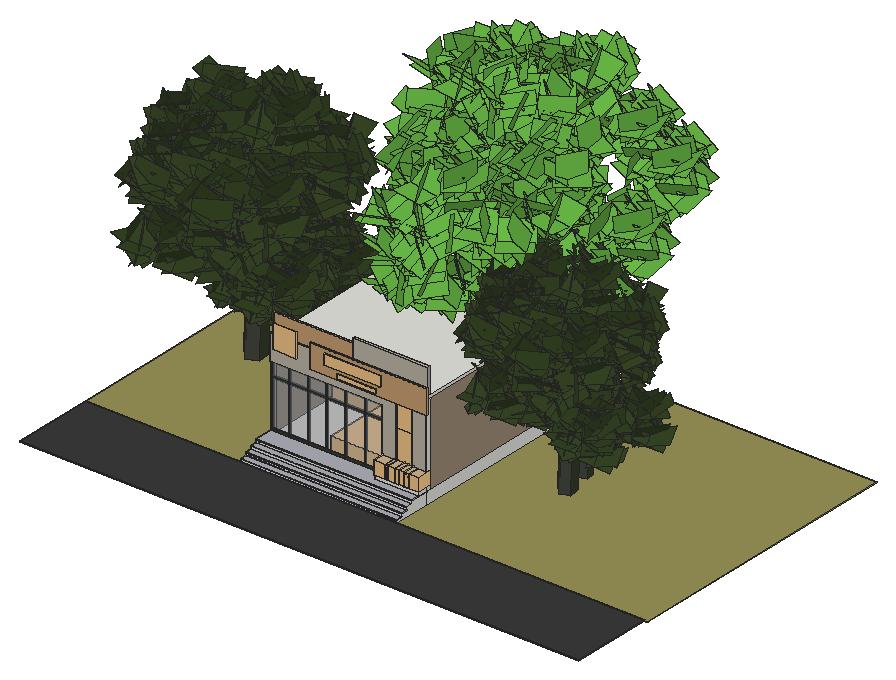
# SketchUp Ruby script. Lengths in inches.
U = 1.inch
M = Sketchup.active_model
def pt(a) = Geom::Point3d.new(a.map { |v| v * U })
def face(e, loops, mat)
  f = e.add_face(loops[0].map { |a| pt(a) })
  loops[1..].each { |l| e.add_face(l.map { |a| pt(a) }).erase! }
  f.material = f.back_material = mat if mat
  f
end
# faces: each face lists its corners as indices into pts; further lists are holes
def faces(e, pts, list, mat = nil) = list.each { |f| face(e, (f[0].is_a?(Array) ? f : [f]).map { |l| l.map { |i| pts[i] } }, mat) }
# xy, xz, yz: faces in a plane at the given z, y or x. An outline is a flat list of corners, or four numbers for a rectangle; further outlines are holes
def ring(l) = l.size == 4 ? [[l[0], l[1]], [l[2], l[1]], [l[2], l[3]], [l[0], l[3]]] : l.each_slice(2).to_a
def flat(e, list, mat, &to3) = list.each { |f| face(e, (f[0].is_a?(Array) ? f : [f]).map { |l| ring(l).map { |u, v| to3.(u, v) } }, mat) }
def xy(e, z, list, mat = nil) = flat(e, list, mat) { |x, y| [x, y, z] }
def xz(e, y, list, mat = nil) = flat(e, list, mat) { |x, z| [x, y, z] }
def yz(e, x, list, mat = nil) = flat(e, list, mat) { |y, z| [x, y, z] }
def lines(e, pts, list) = list.each { |a, b| e.add_line(pt(pts[a]), pt(pts[b])) }
# prism: a flat outline (further loops are holes) pulled along v
def prism(e, loops, v, mat = nil)
  f = face(e, loops, mat); d = Geom::Vector3d.new(v.map { |x| x * U })
  f.pushpull(f.normal.samedirection?(d) ? d.length : -d.length)
end
def box(e, o, s, mat = nil) = prism(e, [[o, [o[0] + s[0], o[1], o[2]], [o[0] + s[0], o[1] + s[1], o[2]], [o[0], o[1] + s[1], o[2]]]], [0, 0, s[2]], mat)
def at(x, y, z, deg = 0) = Geom::Transformation.translation(pt([x, y, z])) * Geom::Transformation.rotation(ORIGIN, Z_AXIS, deg.degrees)
def axes(o, x, y, z) = Geom::Transformation.new([*x, 0, *y, 0, *z, 0, *pt(o).to_a, 1])
def part(name) = M.definitions.add(name)
# library, detail: a bought-in or finely detailed component or shape, given as its bounding box
def library(name, o, s) = part(name).tap { |d| box(d.entities, o, s) }
def detail(e, o, s) = box(e.add_group.entities, o, s)
def put(e, d, t, mat = nil) = e.add_instance(d, t).tap { |i| i.material = mat if mat }
def group(e, t, mat = nil) = e.add_group.tap { |g| g.transformation = t; g.material = mat if mat }.entities
root = M.entities
M.materials.add("Concrete_06_1K").color = [183, 176, 162]
M.materials.add("Glass_Basic_01").color = [161, 173, 186]
M.materials["Glass_Basic_01"].alpha = 0.25
M.materials.add("LondonPlane").color = [106, 186, 71]
M.materials.add("M02_Ash_Whisper").color = [196, 196, 196]
M.materials.add("M07_Charcoal_Gleam").color = [58, 58, 58]
M.materials.add("Marble_01_1K").color = [230, 221, 211]
M.materials.add("Marble_07_1K").color = [36, 34, 36]
M.materials.add("Marble_20_1K").color = [172, 173, 182]
M.materials.add("OakLeaves").color = [53, 68, 35]
M.materials.add("Plaster_02_1K").color = [157, 140, 119]
M.materials.add("Soil_04_1K").color = [152, 146, 88]
M.materials.add("TreeBark").color = [59, 61, 54]
M.materials.add("Wood_Veneer_15_1K").color = [193, 154, 111]
M.materials.add("[Color B06]").color = [178, 70, 33]
c1 = library("TOASTED",[-0.01,0,0],[55.46,9.9,1])
c2 = library("TOAST & COFFEE",[-0.01,0,0],[101.64,9.9,1])
c3 = part("Leaves1\#1")
xy(c3.entities,0,[[0,0,18.9,13.83]],"OakLeaves")
c4 = part("Leaves3\#1")
put(c4.entities,c3,axes([5.03,0,3.17],[0.83485,0,0.55048],[0,1,0],[-0.55048,0,0.83485]))
put(c4.entities,c3,at(0,0.43,5.55))
put(c4.entities,c3,axes([1.03,1.26,13.36],[0.83485,0.53172,0.14247],[0,0.25882,-0.96593],[-0.55048,0.8064,0.21607]))
c5 = part("Leaves9\#1")
put(c5.entities,c4,at(0,20.48,0))
put(c5.entities,c4,axes([31.13,19.18,5.89],[-0.4626,-0.37946,0.80126],[-0.18973,0.92521,0.32862],[-0.86603,0,-0.5]))
put(c5.entities,c4,at(4.73,14.72,5.55,-45))
c6 = part("LeavesLarge\#1")
put(c6.entities,c5,axes([12.5,27.63,8.89],[1.36,0,0],[0,1.36,0],[0,0,1.36]))
put(c6.entities,c5,axes([17.32,3.99,13.67],[1.26537,0.49844,0],[-0.49844,1.26537,0],[0,0,1.36]))
put(c6.entities,c5,axes([11.69,23.63,-12.83],[1.36,0,0],[0,1.21284,0.61531],[0,-0.61531,1.21284]))
c7 = part("Branch")
xy(c7.entities,0,[[5.71,0,0,7.86,5.71,15.73,14.96,12.72,14.96,3]],"TreeBark")
xy(c7.entities,87.8,[[6.44,2.25,13.05,4.39,13.05,11.33,6.44,13.48,2.36,7.86]],"TreeBark")
yz(c7.entities,14.96,[[3,0,12.72,46.46]],"TreeBark")
p = [[0,7.86,0],[5.71,0,0],[5.71,0,46.46],[0,7.86,46.46],[14.96,3,0],[14.96,3,46.46],
  [5.71,15.73,0],[5.71,15.73,46.46],[14.96,12.72,0],[14.96,12.72,46.46],[2.36,7.86,87.8],[6.44,2.25,87.8],
  [13.05,4.39,87.8],[13.05,11.33,87.8],[6.44,13.48,87.8]]
faces(c7.entities,p,[[0,1,2,3],[1,4,5,2],[6,0,3,7],[8,6,7,9],[10,3,2,11],[5,12,11,2],[9,13,12,5],[3,10,14,7],
  [7,14,13,9]],"TreeBark")
c8 = part("VeryLargeGroup\#1")
put(c8.entities,c6,at(173.76,146.72,70.08,102.9))
put(c8.entities,c6,at(132.27,106.75,136.73,42.9))
put(c8.entities,c6,at(131.49,50.64,119.21,42.9))
put(c8.entities,c6,at(70.65,58.78,97.86,42.9))
put(c8.entities,c6,at(195.71,86.26,134.76,102.9))
put(c8.entities,c6,at(196.25,96.99,71.2,102.9))
put(c8.entities,c6,at(144.95,113.53,160.58,102.9))
put(c8.entities,c6,at(103.63,52.73,72.72,102.9))
put(c8.entities,c6,at(95.79,82.96,122.8,42.9))
put(c8.entities,c6,at(121.16,40.64,113.49))
put(c8.entities,c6,at(65.4,87.38,150.56,42.9))
c9 = part("Oak Tree\#1")
put(c9.entities,c6,axes([113.07,95,108.63],[0.62266,0.60584,0],[-0.57861,0.65196,0],[0,0,1]))
put(c9.entities,c6,axes([147.33,45.07,91.12],[0.62266,0.60584,0],[-0.57861,0.65196,0],[0,0,1]))
put(c9.entities,c7,axes([78.54,84.74,5.12],[0.85,0,0],[0,0.89,0],[0,0,0.68]))
put(c9.entities,c7,axes([80.98,86.82,60.25],[0.49449,0.06108,0.20312],[0.03062,0.48749,-0.28823],[-0.25331,0.3542,0.71905]))
put(c9.entities,c6,axes([112.41,45.07,91.12],[0.62266,0.60584,0],[-0.57861,0.65196,0],[0,0,1]))
put(c9.entities,c7,axes([83.0625,90.37,65.57],[0.04738,-0.40054,-0.42279],[0.33578,0.31351,-0.3229],[0.56881,-0.30161,0.44897]))
put(c9.entities,c6,axes([52.92,85.06,122.46],[0.62266,0.60584,0],[-0.57861,0.65196,0],[0,0,1]))
put(c9.entities,c7,axes([135.51,66.7,99.02],[-0.10237,-0.10566,-0.12322],[0.14217,-0.06826,-0.09646],[0.01884,-0.30818,0.30456]))
put(c9.entities,c7,axes([134.01,64.3,100.08],[0.05377,-0.0892,-0.1105],[0.04609,0.11327,-0.08439],[0.26984,-0.00818,0.19009]))
put(c9.entities,c7,axes([108.98,74.71,83.27],[-0.0456,-0.14333,-0.17519],[0.205,-0.00584,-0.07891],[0.06355,-0.37509,0.34064]))
put(c9.entities,c8,axes([166.9,196.22,-17],[-0.84867,0.04968,0],[-0.04745,-0.88861,0],[0,0,1]))
put(c9.entities,c7,axes([115.72,70.28,87.99],[0.13572,-0.08151,-0.17161],[-0.01536,0.19053,-0.13106],[0.37604,0.1941,0.29522]))
put(c9.entities,c6,axes([82.07,73.83,94.71],[0.62266,0.60584,0],[-0.57861,0.65196,0],[0,0,1]))
put(c9.entities,c6,axes([49.9,103.37,128.83],[0.85,0,0],[0,0.89,0],[0,0,1]))
put(c9.entities,c6,axes([60.69,52.32,69.77],[0.62266,0.60584,0],[-0.57861,0.65196,0],[0,0,1]))
put(c9.entities,c8,axes([-32.96,76.23,-14.92],[0.63365,-0.59321,0],[0.56655,0.66347,0],[0,0,1]))
put(c9.entities,c6,axes([148.74,43.73,62.32],[0.62266,0.60584,0],[-0.57861,0.65196,0],[0,0,1]))
put(c9.entities,c6,axes([171.77,28.54,106.66],[-0.18976,0.86754,0],[-0.82855,-0.19869,0],[0,0,1]))
put(c9.entities,c6,axes([123.85,107.35,132.49],[-0.18976,0.86754,0],[-0.82855,-0.19869,0],[0,0,1]))
put(c9.entities,c7,axes([68.3125,110.27,106.91],[0.16551,-0.09941,-0.20928],[-0.01873,0.23235,-0.15983],[0.45859,0.2367,0.36003]))
put(c9.entities,c7,axes([63.14,120.64,123.64],[-0.09701,0.1208,-0.16533],[-0.04635,-0.1777,-0.12627],[-0.40159,-0.04524,0.28442]))
put(c9.entities,c7,axes([74.24,101.99,91.19],[-0.06262,0.18872,-0.20928],[-0.13145,-0.18822,-0.15983],[-0.49441,0.13638,0.36003]))
put(c9.entities,c7,axes([96.64,125.8125,125.76],[-0.11632,0.09819,-0.06186],[-0.1008,-0.12782,0.00621],[-0.12813,0.13396,0.60191]))
put(c9.entities,c7,axes([65.72,120.76,123.43],[-0.06648,0.05611,-0.03535],[-0.0576,-0.07304,0.00355],[-0.07323,0.07655,0.34397]))
put(c9.entities,c6,axes([113.16,46.93,44.625],[-0.18976,0.86754,0],[-0.82855,-0.19869,0],[0,0,1]))
put(c9.entities,c6,axes([167.45,86.32,43.11],[-0.18976,0.86754,0],[-0.82855,-0.19869,0],[0,0,1]))
put(c9.entities,c6,axes([146.75,14.09,79.13],[0.62266,0.60584,0],[-0.57861,0.65196,0],[0,0,1]))
c10 = part("OakTree")
put(c10.entities,c9,axes([-90.62,-63.01,26.91],[1.2322,0,0],[0,1.2322,0],[0,0,1.2322]))
c11 = part("Leaves1")
xy(c11.entities,0,[[0,0,13.85,13.83]],"LondonPlane")
c12 = part("Leaves3")
put(c12.entities,c11,axes([5.03,0,3.17],[0.83485,0,0.55048],[0,1,0],[-0.55048,0,0.83485]))
put(c12.entities,c11,at(0,0.43,5.55))
put(c12.entities,c11,axes([1.03,1.26,13.36],[0.83485,0.53172,0.14247],[0,0.25882,-0.96593],[-0.55048,0.8064,0.21607]))
c13 = part("Leaves9")
put(c13.entities,c12,at(0,20.48,0))
put(c13.entities,c12,axes([31.13,19.18,5.89],[-0.4626,-0.37946,0.80126],[-0.18973,0.92521,0.32862],[-0.86603,0,-0.5]))
put(c13.entities,c12,at(4.73,14.72,5.55,-45))
c14 = part("LeavesLarge")
put(c14.entities,c13,axes([12.5,27.63,8.89],[1.36,0,0],[0,1.36,0],[0,0,1.36]))
put(c14.entities,c13,axes([17.32,3.99,13.67],[1.26537,0.49844,0],[-0.49844,1.26537,0],[0,0,1.36]))
put(c14.entities,c13,axes([11.69,23.63,-12.83],[1.36,0,0],[0,1.21284,0.61531],[0,-0.61531,1.21284]))
c15 = part("Branch\#1")
xy(c15.entities,0,[[5.71,-1.15,-0.84,7.86,5.71,17.17,15.52,14.46,15.8,1.85]],"TreeBark")
xy(c15.entities,9.15,[[5.71,0,0,7.86,5.71,15.73,14.96,12.72,14.96,3]])
xy(c15.entities,87.8,[[6.44,2.25,13.05,4.39,13.05,11.33,6.44,13.48,2.36,7.86]],"TreeBark")
yz(c15.entities,14.96,[[3,9.15,12.72,46.46]],"TreeBark")
p = [[-0.84,7.86,0],[5.71,-1.15,0],[0,7.86,9.15],[5.71,0,9.15],[15.8,1.85,0],[14.96,3,9.15],
  [15.52,14.46,0],[14.96,12.72,9.15],[5.71,15.73,9.15],[5.71,17.17,0],[0,7.86,46.46],[5.71,0,46.46],
  [14.96,3,46.46],[5.71,15.73,46.46],[14.96,12.72,46.46],[2.36,7.86,87.8],[6.44,2.25,87.8],[13.05,4.39,87.8],
  [13.05,11.33,87.8],[6.44,13.48,87.8]]
faces(c15.entities,p,[[0,1,2],[3,2,1],[1,4,3],[5,3,4],[4,6,5],[7,5,6],[2,8,0],[9,0,8],
  [8,7,9],[6,9,7],[10,2,3,11],[11,3,5,12],[13,8,2,10],[14,7,8,13],[15,10,11,16],[12,17,16,11],
  [14,18,17,12],[10,15,19,13],[13,19,18,14]],"TreeBark")
c16 = part("VeryLargeGroup")
put(c16.entities,c14,at(173.76,146.72,70.08,102.9))
put(c16.entities,c14,at(132.27,106.75,136.73,42.9))
put(c16.entities,c14,at(131.49,50.64,119.21,42.9))
put(c16.entities,c14,at(70.65,58.78,97.86,42.9))
put(c16.entities,c14,at(195.71,86.26,134.76,102.9))
put(c16.entities,c14,at(144.95,113.53,160.58,102.9))
put(c16.entities,c14,at(95.79,82.96,122.8,42.9))
put(c16.entities,c14,at(121.16,40.64,113.49))
put(c16.entities,c14,at(65.4,87.38,150.56,42.9))
c17 = part("Oak Tree")
put(c17.entities,c14,axes([256.375,199.39,203.5625],[1.41181,1.2715,0],[-1.31194,1.3683,0],[0,0,1.87387]))
put(c17.entities,c14,axes([334.0625,94.58,170.74],[1.41181,1.2715,0],[-1.31194,1.3683,0],[0,0,1.87387]))
put(c17.entities,c15,axes([181.48,185.6,-12.47],[1.23808,0,0],[0,1.19992,0],[0,0,1.4767]))
put(c17.entities,c7,axes([185.6875,187.125,114.14],[0.77239,0.0883,0.26221],[0.04783,0.70483,-0.37208],[-0.39567,0.5121,0.92823]))
put(c17.entities,c14,axes([254.875,94.58,170.74],[1.41181,1.2715,0],[-1.31194,1.3683,0],[0,0,1.87387]))
put(c17.entities,c7,axes([185.54,194.07,115.44],[0.30328,-0.52119,-0.39208],[0.59636,0.40795,-0.08887],[0.43168,-0.39246,0.85154]))
put(c17.entities,c14,axes([120,178.52,229.48],[1.41181,1.2715,0],[-1.31194,1.3683,0],[0,0,1.87387]))
put(c17.entities,c16,axes([378.43,411.8125,-31.85],[-1.92427,0.10427,0],[-0.10758,-1.86496,0],[0,0,1.87387]))
put(c17.entities,c14,axes([186.08,154.95,177.47],[1.41181,1.2715,0],[-1.31194,1.3683,0],[0,0,1.87387]))
put(c17.entities,c14,axes([113.14,216.94,241.4],[1.92728,0,0],[0,1.86788,0],[0,0,1.87387]))
put(c17.entities,c14,axes([137.61,109.8,130.73],[1.41181,1.2715,0],[-1.31194,1.3683,0],[0,0,1.87387]))
put(c17.entities,c14,axes([367.74,59.89,199.875],[-0.43026,1.82073,0],[-1.87864,-0.417,0],[0,0,1.87387]))
put(c17.entities,c14,axes([280.8125,225.29,248.27],[-0.43026,1.82073,0],[-1.87864,-0.417,0],[0,0,1.87387]))
put(c17.entities,c7,axes([157.09,232.74,192.91],[0.2801,0.02039,0.27837],[0.09318,0.35928,-0.12043],[-0.58565,0.34803,0.60033]))
put(c17.entities,c7,axes([159.97,234.64,194.38],[0.24034,0.2343,-0.30981],[-0.37841,0.08329,-0.23661],[-0.14761,0.90353,0.53297]))
put(c17.entities,c7,axes([211.65,171.01,145.95],[-0.03711,0.11776,0.1604],[0.03079,-0.1533,0.1271],[0.66418,0.16067,0.04347]))
put(c17.entities,c14,axes([256.58,98.5,83.62],[-0.43026,1.82073,0],[-1.87864,-0.417,0],[0,0,1.87387]))
put(c17.entities,c14,axes([332.74,29.57,148.28],[1.41181,1.2715,0],[-1.31194,1.3683,0],[0,0,1.87387]))
put(c17.entities,c7,axes([227.6,154.4,186.34],[0.12193,-0.18721,-0.20706],[0.10449,0.23771,-0.15814],[0.61184,-0.01717,0.35621]))
put(c17.entities,c7,axes([209.13,115.3,167.91],[0.2745,-0.00506,-0.13197],[-0.12719,-0.0592,-0.26973],[-0.04219,0.69189,-0.14502]))
put(c17.entities,c14,axes([297.36,115.57,144.59],[-0.42387,1.81941,0],[-1.87991,-0.4236,0],[0,0,1.87387]))
put(c17.entities,c14,axes([337.59,114.82,111.03],[-0.42387,1.81941,0],[-1.87991,-0.4236,0],[0,0,1.87387]))
put(c17.entities,c14,axes([224.75,92.43,153.38],[-0.42387,1.81941,0],[-1.87991,-0.4236,0],[0,0,1.87387]))
put(c17.entities,c14,axes([237.98,297.99,190.71],[-0.43026,1.82073,0],[-1.87864,-0.417,0],[0,0,1.87387]))
put(c17.entities,c14,axes([199,174.74,83.62],[0.4654,1.81207,0],[-1.85717,0.50406,0],[0,0,1.87387]))
put(c17.entities,c7,axes([172.5,215.12,158.46],[-0.04397,0.1628,-0.21774],[-0.10146,-0.21192,-0.14955],[-0.75806,0.2221,0.19842]))
put(c17.entities,c14,axes([288.12,208.82,172.43],[1.41181,1.2715,0],[-1.31194,1.3683,0],[0,0,1.87387]))
put(c17.entities,c16,axes([-154.51,140.25,-34.86],[1.41308,-1.31031,0],[1.27495,1.36535,0],[0,0,1.87387]))
c18 = part("Beech")
put(c18.entities,c17,at(-171.79,-49.38,-9.59))
c19 = part("Group\#2")
box(c19.entities,[0,0,0],[2,2,114])
c20 = part("Group\#19")
box(c20.entities,[0,0,0],[300,13,1])
c21 = library("Group\#20",[0,0,0],[44,178,2])
c22 = library("Group\#23",[0,0,0],[45.92,1,45.67])
c23 = library("Group\#40",[0,0,0],[160.51,127.83,29.04])
c24 = library("Group\#43",[-0.5625,-0.42,-0.74],[14.57,14.83,12.98])
put(root,c1,axes([523.1,222.47,152.37],[1.9602,0,0],[0,0,1.9602],[0,-1.9602,0]),"M02_Ash_Whisper")
put(root,c2,axes([547.59,222.47,137.39],[0.73,0,0],[0,0,0.73],[0,-0.73,0]),"M02_Ash_Whisper")
put(root,c10,axes([918.125,459.66,-94.53],[-1.5971,0.87795,-0.01063],[-0.87793,-1.59652,0.04497],[0.01236,0.04453,1.82195]))
put(root,c18,axes([588.74,346.96,3.54],[1.64236,0,0],[0,1.64236,0],[0,0,1.64236]))
put(root,c10,axes([308.67,506.51,-103.9375],[-1.95996,1.07742,-0.01304],[-1.07739,-1.95924,0.05519],[0.0141,0.05082,2.07939]))
put(root,c10,axes([332.41,498.16,-77.67],[-1.21831,0.66972,-0.00811],[-0.66971,-1.21787,0.03431],[0.00877,0.03159,1.29255]))
put(root,c10,axes([893.12,498.16,-77.67],[-1.21831,0.66972,-0.00811],[-0.66971,-1.21787,0.03431],[0.00877,0.03159,1.29255]))
g1 = group(root,at(415.13,228.47,0),"M07_Charcoal_Gleam")
g2 = group(g1,at(0,0,0))
prism(g2,[[[0,0,0],[216,0,0],[216,0,120],[0,0,120]],[[3,0,117],[213,0,117],[213,0,3],[3,0,3]]],[0,3,0])
g3 = group(g1,at(3,1.5,3),"Glass_Basic_01")
box(g3,[0,0,0],[210,1,114])
put(g1,c19,at(180,0.5,3))
put(g1,c19,at(106,0.5,3))
put(g1,c19,at(70,0.5,3))
g4 = group(g1,at(3,0,90))
box(g4,[0,0,0],[210,3,3])
put(g1,c19,at(142,0.5,3))
put(g1,c19,at(34,0.5,3))
g5 = group(root,at(415.13,237.47,0))
xy(g5,0,[[216,-9,300,0]])
xy(g5,120,[[0,-9,216,0]])
xy(g5,156,[[0,-9,300,0]])
xz(g5,-9,[[216,0,243,0,243,156,0,156,0,120,216,120],[273,0,300,156]])
xz(g5,-9,[[243,0,273,156]],"[Color B06]")
xz(g5,0,[[216,0,216,120,0,120,0,156,300,156,300,0]])
yz(g5,0,[[-9,120,0,156]])
yz(g5,216,[[-9,0,0,120]])
yz(g5,300,[[-9,0,0,156]])
g6 = group(root,at(706.13,237.47,0),"Plaster_02_1K")
box(g6,[0,0,0],[9,287.68,156])
g7 = group(root,at(415.13,237.47,0),"Plaster_02_1K")
box(g7,[0,-6,0],[9,293.68,156])
g8 = group(root,at(415.13,534.15,0,-90),"Plaster_02_1K")
box(g8,[0,0,0],[9,300,156])
g9 = group(root,at(415.13,228.47,156))
box(g9,[0,0,0],[300,305.68,6])
g10 = group(root,at(571.13,229.97,162),"Concrete_06_1K")
box(g10,[0,0,0],[144,6,49.67])
g11 = group(root,at(415.13,225.47,0),"Concrete_06_1K")
prism(g11,[[[243,3,168],[243,3,0],[216,3,0],[216,3,120],[0,3,120],[0,3,168]]],[0,-3,0])
g12 = group(root,at(688.13,225.47,0),"Concrete_06_1K")
box(g12,[0,0,0],[27,3,162])
g13 = group(root,at(596.44,222.47,79.93),"Wood_Veneer_15_1K")
xy(g13,53.89,[[-102.72,0,123.19,3]])
xy(g13,100.07,[[-102.72,0,123.19,3]])
xz(g13,0,[[-102.72,53.89,123.19,100.07]],"Wood_Veneer_15_1K")
xz(g13,3,[[-102.72,53.89,123.19,100.07]])
yz(g13,-102.72,[[0,53.89,3,100.07]])
yz(g13,123.19,[[0,53.89,3,100.07]])
g14 = group(root,at(497.33,235.97,117.11),"Wood_Veneer_15_1K")
xy(g14,44.89,[[-82.2,0,123.19,3]])
xy(g14,82.56,[[-82.2,0,123.19,3]])
xz(g14,0,[[-82.2,44.89,123.19,82.56]],"Wood_Veneer_15_1K")
xz(g14,3,[[-82.2,44.89,123.19,82.56]])
yz(g14,-82.2,[[0,44.89,3,82.56]])
yz(g14,123.19,[[0,44.89,3,82.56]])
g15 = group(root,at(415.13,228.47,-12))
xy(g15,-12,[[0,0,300,305.68]])
xy(g15,12,[[0,0,300,305.68]],"Marble_01_1K")
xz(g15,0,[[0,-12,300,12]])
xz(g15,305.68,[[0,-12,300,12]])
yz(g15,0,[[0,-12,305.68,12]])
yz(g15,300,[[0,-12,305.68,12]])
g16 = group(root,at(415.13,156.47,-24))
prism(g16,[[[0,72,23],[0,72,0],[0,0,0],[0,0,5],[0,12,5],[0,12,11],[0,24,11],[0,24,17],[0,36,17],[0,36,23]]],[300,0,0])
put(root,c20,at(415.13,155.47,-19),"Marble_20_1K")
put(root,c20,at(415.13,167.47,-13),"Marble_20_1K")
put(root,c20,at(415.13,179.47,-7),"Marble_20_1K")
g17 = group(root,at(415.13,215.47,-1),"Marble_20_1K")
box(g17,[0,-24,0],[300,37,1])
put(root,c21,axes([658.13,228.47,88.43],[0.68182,0,0],[0,0,0.49958],[0,-0.88,0]))
put(root,c21,axes([658.13,228.47,0],[0.68182,0,0],[0,0,0.49958],[0,-0.88,0]))
put(root,c22,at(421.17,224.47,141.86))
g18 = group(root,at(116.67,156.47,-25),"Soil_04_1K")
box(g18,[0,0,0],[1080.73,547.46,1])
g19 = group(root,at(116.67,0,-25),"M07_Charcoal_Gleam")
box(g19,[0,0,0],[1073.18,156.47,1],"M07_Charcoal_Gleam")
put(root,c23,at(529.81,229.97,0))
put(root,c23,at(430,356.97,0))
g20 = group(root,at(631.13,208.09,0))
xy(g20,0,[[0,0,84,17.38]])
xy(g20,14,[[2.5,2.5,81.5,14.88]],"Soil_04_1K")
xy(g20,15,[[[0,0,84,17.38],[2.5,2.5,81.5,14.88]]])
xz(g20,0,[[0,0,84,15]])
xz(g20,2.5,[[2.5,14,81.5,15]])
xz(g20,14.88,[[2.5,14,81.5,15]])
xz(g20,17.38,[[0,0,84,15]])
yz(g20,0,[[0,0,17.38,15]])
yz(g20,2.5,[[2.5,14,14.88,15]])
yz(g20,81.5,[[2.5,14,14.88,15]])
yz(g20,84,[[0,0,17.38,15]])
g21 = group(root,at(630.13,207.09,15),"Marble_07_1K")
prism(g21,[[[0,0,0],[0,18.38,0],[86,18.38,0],[86,0,0]],[[82.5,3.5,0],[82.5,15.88,0],[3.5,15.88,0],[3.5,3.5,0]]],[0,0,1])
put(root,c24,axes([633.48,203.8,11.61],[1.887,0,0],[0,1.887,0],[0,0,1.887]))
put(root,c24,axes([654.82,203.8,11.61],[1.887,0,0],[0,1.887,0],[0,0,1.887]))
put(root,c24,axes([692.34,203.8,11.61],[1.887,0,0],[0,1.887,0],[0,0,1.887]))
put(root,c24,axes([673.91,203.8,11.61],[1.887,0,0],[0,1.887,0],[0,0,1.887]))
